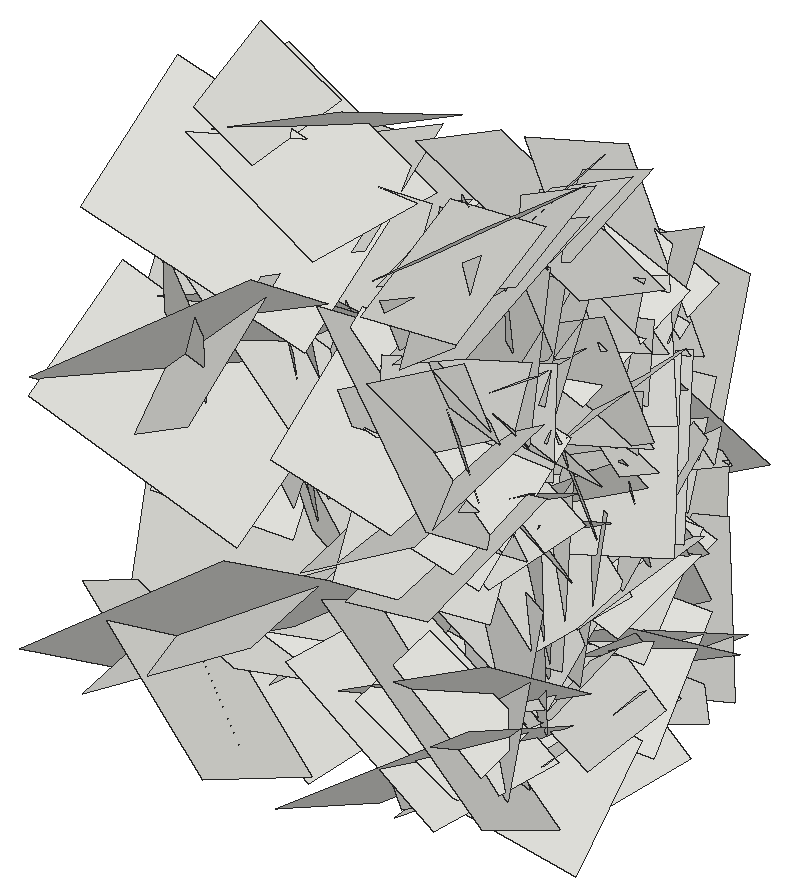
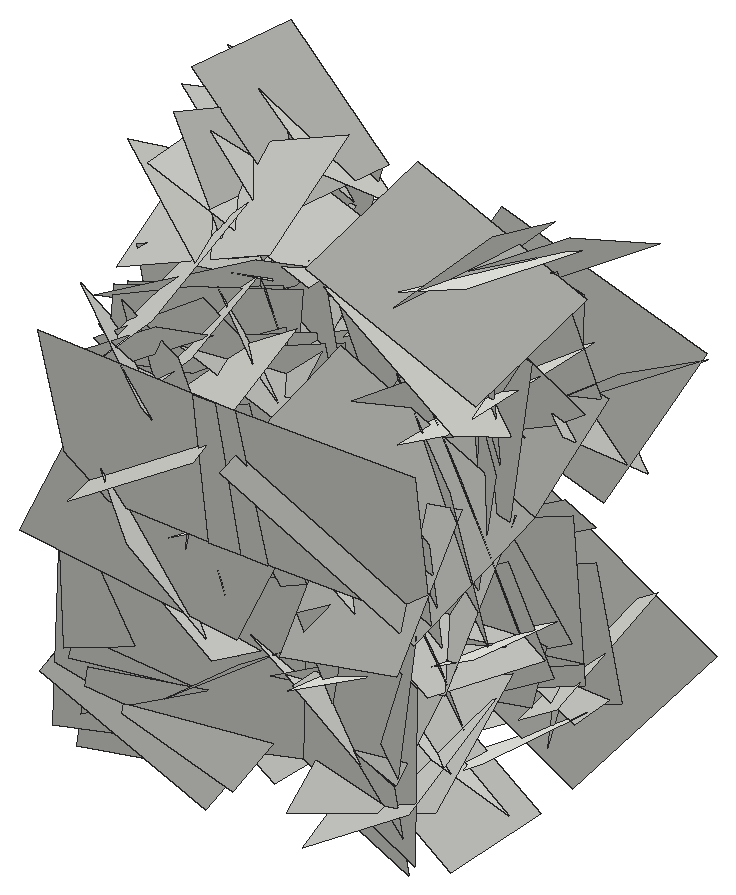
# SketchUp Ruby script. Lengths in inches.
U = 1.inch
M = Sketchup.active_model
def pt(a) = Geom::Point3d.new(a.map { |v| v * U })
def face(e, loops, mat)
  f = e.add_face(loops[0].map { |a| pt(a) })
  loops[1..].each { |l| e.add_face(l.map { |a| pt(a) }).erase! }
  f.material = f.back_material = mat if mat
  f
end
# faces: each face lists its corners as indices into pts; further lists are holes
def faces(e, pts, list, mat = nil) = list.each { |f| face(e, (f[0].is_a?(Array) ? f : [f]).map { |l| l.map { |i| pts[i] } }, mat) }
# xy, xz, yz: faces in a plane at the given z, y or x. An outline is a flat list of corners, or four numbers for a rectangle; further outlines are holes
def ring(l) = l.size == 4 ? [[l[0], l[1]], [l[2], l[1]], [l[2], l[3]], [l[0], l[3]]] : l.each_slice(2).to_a
def flat(e, list, mat, &to3) = list.each { |f| face(e, (f[0].is_a?(Array) ? f : [f]).map { |l| ring(l).map { |u, v| to3.(u, v) } }, mat) }
def xy(e, z, list, mat = nil) = flat(e, list, mat) { |x, y| [x, y, z] }
def xz(e, y, list, mat = nil) = flat(e, list, mat) { |x, z| [x, y, z] }
def yz(e, x, list, mat = nil) = flat(e, list, mat) { |y, z| [x, y, z] }
def lines(e, pts, list) = list.each { |a, b| e.add_line(pt(pts[a]), pt(pts[b])) }
# prism: a flat outline (further loops are holes) pulled along v
def prism(e, loops, v, mat = nil)
  f = face(e, loops, mat); d = Geom::Vector3d.new(v.map { |x| x * U })
  f.pushpull(f.normal.samedirection?(d) ? d.length : -d.length)
end
def box(e, o, s, mat = nil) = prism(e, [[o, [o[0] + s[0], o[1], o[2]], [o[0] + s[0], o[1] + s[1], o[2]], [o[0], o[1] + s[1], o[2]]]], [0, 0, s[2]], mat)
def at(x, y, z, deg = 0) = Geom::Transformation.translation(pt([x, y, z])) * Geom::Transformation.rotation(ORIGIN, Z_AXIS, deg.degrees)
def axes(o, x, y, z) = Geom::Transformation.new([*x, 0, *y, 0, *z, 0, *pt(o).to_a, 1])
def part(name) = M.definitions.add(name)
# library, detail: a bought-in or finely detailed component or shape, given as its bounding box
def library(name, o, s) = part(name).tap { |d| box(d.entities, o, s) }
def detail(e, o, s) = box(e.add_group.entities, o, s)
def put(e, d, t, mat = nil) = e.add_instance(d, t).tap { |i| i.material = mat if mat }
def group(e, t, mat = nil) = e.add_group.tap { |g| g.transformation = t; g.material = mat if mat }.entities
root = M.entities
c1 = part("Component\#6")
p = [[0.01,0,0],[0,3.24,4.54],[4.32,3.24,4.54],[4.33,0,0]]
faces(c1.entities,p,[[0,1,2,3]])
put(root,c1,axes([410.71,200.85,29.625],[-0.04324,0.39016,0.69087],[-0.10275,0.68414,-0.39209],[0.83473,0.10443,-0.01247]))
put(root,c1,axes([404.88,202.49,32.61],[0.11645,-0.17214,0.59947],[0.01233,0.60916,0.17278],[-0.661,-0.01896,0.10883]))
put(root,c1,axes([410.71,202.49,32.61],[-0.11645,-0.17214,0.59947],[-0.01233,0.60916,0.17278],[0.661,-0.01896,0.10883]))
put(root,c1,axes([400.91,199.54,32.72],[-0.14681,1.15124,0.44909],[-0.05729,0.44582,-1.15954],[1.30862,0.14867,-0.00039]))
put(root,c1,axes([414.68,199.54,32.72],[0.14681,1.15124,0.44909],[0.05729,0.44582,-1.15954],[-1.30862,0.14867,-0.00039]))
put(root,c1,axes([400.91,206.55,33.15],[0.00164,-0.95203,-0.71322],[-0.09471,-0.7113,0.94927],[1.25737,-0.05234,0.07244]))
put(root,c1,axes([414.68,206.55,33.15],[-0.00164,-0.95203,-0.71322],[0.09471,-0.7113,0.94927],[-1.25737,-0.05234,0.07244]))
put(root,c1,axes([410.71,202.42,34.22],[-0.03507,0.56649,-0.26791],[0.06705,-0.26389,-0.56581],[0.66085,0.05684,0.04319]))
put(root,c1,axes([410.71,205,37.54],[0.1597,-0.46751,-0.41946],[-0.05532,-0.43919,0.47075],[0.66349,0.07592,0.14021]))
put(root,c1,axes([400.91,204.59,30.02],[-0.04301,-1.09683,0.72238],[-0.12053,0.72294,1.0913],[1.38692,0.02882,0.11724]))
put(root,c1,axes([414.68,204.59,30.02],[0.04301,-1.09683,0.72238],[0.12053,0.72294,1.0913],[-1.38692,0.02882,0.11724]))
put(root,c1,axes([410.71,201.89,25.36],[0.12511,0.60489,0.30184],[-0.04372,0.31228,-0.60968],[0.71524,-0.08672,-0.09007]))
put(root,c1,axes([400.91,201.95,25.76],[0.02109,1.10253,-0.4508],[-0.04504,-0.44992,-1.10225],[1.2618,-0.03449,-0.03181]))
put(root,c1,axes([414.68,201.95,25.76],[-0.02109,1.10253,-0.4508],[0.04504,-0.44992,-1.10225],[-1.2618,-0.03449,-0.03181]))
put(root,c1,axes([414.68,200.125,30.08],[0.25415,0.9144,0.59243],[0.00684,0.60541,-0.93704],[-1.1549,0.20481,0.12483]))
put(root,c1,axes([400.91,205.99,22.98],[0.14358,-1.11124,-0.06865],[0.09474,-0.05808,1.11649],[1.17635,0.14031,-0.08154]))
put(root,c1,axes([414.68,205.99,22.98],[-0.14358,-1.11124,-0.06865],[-0.09474,-0.05808,1.11649],[-1.17635,0.14031,-0.08154]))
put(root,c1,axes([400.91,206.07,20.81],[-0.31441,-1.20333,0.63493],[-0.01893,0.65323,1.22967],[1.44208,-0.25378,0.15457]))
put(root,c1,axes([414.68,206.07,20.81],[0.31441,-1.20333,0.63493],[0.01893,0.65323,1.22967],[-1.44208,-0.25378,0.15457]))
put(root,c1,axes([414.68,201.41,38.375],[0.12316,0.77538,0.57304],[-0.12545,0.58429,-0.76661],[-1.01427,0.02189,0.1644]))
put(root,c1,axes([410.71,204.22,36.67],[0.08595,0.41822,-0.43473],[-0.01861,-0.43682,-0.42351],[0.63917,-0.06896,0.04613]))
put(root,c1,axes([410.71,204.95,35.05],[0.03568,0.1968,-0.61743],[-0.04358,-0.61637,-0.1987],[0.68554,-0.04943,0.01951]))
put(root,c1,axes([414.68,202.75,27.49],[0.17368,0.85862,-0.51485],[-0.1903,-0.48804,-0.87105],[-1.04401,0.2318,0.07312]))
put(root,c1,axes([410.71,202.89,32.22],[-0.0211,0.0618,0.84202],[-0.01452,0.84212,-0.06213],[0.89482,0.01512,0.01885]))
put(root,c1,axes([404.88,203.96,20.97],[-0.02025,-0.24988,0.58047],[0.03388,0.57961,0.25056],[-0.66903,0.03691,-0.00488]))
put(root,c1,axes([410.71,203.96,20.97],[0.02025,-0.24988,0.58047],[-0.03388,0.57961,0.25056],[0.66903,0.03691,-0.00488]))
put(root,c1,axes([410.71,202.23,33.91],[0.02493,0.60398,0.49928],[-0.17768,0.49182,-0.58706],[0.81142,0.08914,-0.14389]))
put(root,c1,axes([410.71,204.33,34.72],[-0.02793,-0.28222,0.66343],[0.05268,0.66158,0.28341],[0.7624,-0.05605,0.00473]))
put(root,c1,axes([414.68,207.21,30.03],[0.00943,-1.01637,-0.0193],[0.00822,-0.01923,1.01638],[-1.07752,-0.00904,0.00758]))
put(root,c1,axes([410.71,207.4,37.82],[-0.14382,-0.92009,0.02073],[-0.06912,0.03051,0.92748],[0.97309,-0.13382,0.06894]))
put(root,c1,axes([414.68,204.65,32.19],[-0.14144,0.68446,-0.34907],[-0.03425,-0.35898,-0.69154],[-0.81371,-0.10387,0.08978]))
put(root,c1,axes([400.91,201.85,37.73],[-0.10519,1.13817,0.58904],[-0.00109,0.59073,-1.14161],[1.35845,0.08861,0.0447]))
put(root,c1,axes([414.68,201.85,37.73],[0.10519,1.13817,0.58904],[0.00109,0.59073,-1.14161],[-1.35845,0.08861,0.0447]))
put(root,c1,axes([404.88,207.84,29.22],[0.13906,-0.51177,-0.49755],[-0.00544,-0.50655,0.51967],[-0.75658,-0.09042,-0.09518]))
put(root,c1,axes([410.71,207.84,29.22],[-0.13906,-0.51177,-0.49755],[0.00544,-0.50655,0.51967],[0.75658,-0.09042,-0.09518]))
put(root,c1,axes([410.71,206.625,39.5],[-0.00312,0.09172,-0.66161],[0.00201,-0.66161,-0.09173],[0.70801,0.00228,-0.00265]))
put(root,c1,axes([414.68,206.58,28.49],[-0.01093,-0.51913,0.63451],[-0.10311,0.63085,0.51456],[-0.86287,-0.06881,-0.06953]))
put(root,c1,axes([414.68,209.72,22.08],[0.18138,-0.91546,-0.54155],[0.07402,-0.53767,0.93095],[-1.12504,-0.18297,-0.02606]))
put(root,c1,axes([400.91,203.71,22.72],[-0.0324,0.32539,1.27516],[0.00551,1.27553,-0.32536],[1.39498,0.00251,0.0309]))
put(root,c1,axes([414.68,203.71,22.72],[0.0324,0.32539,1.27516],[-0.00551,1.27553,-0.32536],[-1.39498,0.00251,0.0309]))
put(root,c1,axes([414.68,204.07,39.0625],[0.02986,0.79051,0.40956],[-0.00815,0.40997,-0.79076],[-0.94369,0.02147,0.01979]))
put(root,c1,axes([400.91,207.91,30.98],[-0.03881,-0.77727,0.6188],[0.26695,0.59174,0.75817],[1.01873,-0.18467,-0.1751]))
put(root,c1,axes([414.68,207.91,30.98],[0.03881,-0.77727,0.6188],[-0.26695,0.59174,0.75817],[-1.01873,-0.18467,-0.1751]))
put(root,c1,axes([414.68,204.65,33.57],[-0.11682,0.36237,1.1463],[-0.15256,1.13885,-0.37385],[-1.26518,-0.17079,-0.06076]))
put(root,c1,axes([400.91,204.65,33.57],[0.11682,0.36237,1.1463],[0.15256,1.13885,-0.37385],[1.26518,-0.17079,-0.06076]))
put(root,c1,axes([400.91,205.05,35.75],[0.23328,1.34713,-0.22992],[0.05022,-0.24027,-1.36238],[1.44774,-0.20874,0.08431]))
put(root,c1,axes([414.68,205.05,35.75],[-0.23328,1.34713,-0.22992],[-0.05022,-0.24027,-1.36238],[-1.44774,-0.20874,0.08431]))
put(root,c1,axes([404.88,206,31.6],[0.1462,-0.08624,0.716],[0.07336,0.72719,0.07426],[-0.76092,0.05354,0.14472]))
put(root,c1,axes([410.71,206,31.6],[-0.1462,-0.08624,0.716],[-0.07336,0.72719,0.07426],[0.76092,0.05354,0.14472]))
put(root,c1,axes([414.68,209.27,26.87],[-0.02942,-0.98917,0.00062],[0.2303,-0.00549,0.9654],[-1.02292,0.02721,0.21733]))
put(root,c1,axes([414.68,205.35,34.65],[-0.12302,0.37909,0.72016],[0.00858,0.72795,-0.38188],[-0.86263,-0.04682,-0.1065]))
put(root,c1,axes([400.91,208.01,36.375],[-0.10923,0.38133,-1.06486],[0.05778,-1.06635,-0.38714],[1.19755,0.08623,-0.07845]))
put(root,c1,axes([414.68,208.01,36.375],[0.10923,0.38133,-1.06486],[-0.05778,-1.06635,-0.38714],[-1.19755,0.08623,-0.07845]))
put(root,c1,axes([414.68,205.67,24.52],[-0.15369,0.87531,0.08009],[0.01982,0.08422,-0.88666],[-0.9315,-0.14262,-0.03208]))
put(root,c1,axes([400.91,209.74,33.23],[0.15201,0.07034,-1.21602],[-0.20156,-1.20811,-0.09231],[1.2753,-0.19933,0.13035]))
put(root,c1,axes([414.68,209.74,33.23],[-0.15201,0.07034,-1.21602],[0.20156,-1.20811,-0.09231],[-1.2753,-0.19933,0.13035]))
put(root,c1,axes([400.91,205.63,39.17],[0.17317,1.06099,0.10432],[0.22006,0.07185,-1.05594],[1.10844,-0.18002,0.19334]))
put(root,c1,axes([414.68,205.63,39.17],[-0.17317,1.06099,0.10432],[-0.22006,0.07185,-1.05594],[-1.10844,-0.18002,0.19334]))
put(root,c1,axes([400.91,205.38,23.16],[0.04798,1.09948,0.05597],[0.01409,0.05547,-1.10036],[1.16688,-0.04588,0.01099]))
put(root,c1,axes([414.68,205.38,23.16],[-0.04798,1.09948,0.05597],[-0.01409,0.05547,-1.10036],[-1.16688,-0.04588,0.01099]))
put(root,c1,axes([404.88,208.95,27.68],[0.1117,0.11156,-0.75397],[0.06454,-0.75994,-0.10393],[-0.80532,-0.04543,-0.11291]))
put(root,c1,axes([410.71,208.95,27.68],[-0.1117,0.11156,-0.75397],[-0.06454,-0.75994,-0.10393],[0.80532,-0.04543,-0.11291]))
put(root,c1,axes([400.91,205.46,24.09],[0.08024,0.04196,1.34674],[-0.06239,1.34768,-0.03868],[1.42687,0.05657,-0.07742]))
put(root,c1,axes([414.68,205.46,24.09],[-0.08024,0.04196,1.34674],[0.06239,1.34768,-0.03868],[-1.42687,0.05657,-0.07742]))
put(root,c1,axes([404.88,210.37,37.54],[0.0852,-0.7988,-0.26142],[0.21653,-0.23617,0.78446],[-0.8642,-0.13792,0.17078]))
put(root,c1,axes([410.71,210.37,37.54],[-0.0852,-0.7988,-0.26142],[-0.21653,-0.23617,0.78446],[0.8642,-0.13792,0.17078]))
put(root,c1,axes([400.91,205.46,33.43],[0.14097,0.63084,0.7943],[-0.06243,0.80455,-0.62912],[1.07339,-0.03606,-0.14091]))
put(root,c1,axes([414.68,205.46,33.43],[-0.14097,0.63084,0.7943],[0.06243,0.80455,-0.62912],[-1.07339,-0.03606,-0.14091]))
put(root,c1,axes([400.91,211.43,33.78],[-0.23599,-0.36182,-1.29322],[-0.09706,-1.30373,0.38052],[1.42014,-0.14923,-0.18889]))
put(root,c1,axes([414.68,211.43,33.78],[0.23599,-0.36182,-1.29322],[0.09706,-1.30373,0.38052],[-1.42014,-0.14923,-0.18889]))
put(root,c1,axes([410.71,206.77,29.69],[0.13468,0.0618,0.68245],[-0.14259,0.68282,-0.03679],[0.71222,0.12502,-0.13642]))
put(root,c1,axes([410.71,209.27,26.93],[0.01951,-0.6006,0.29742],[0.06663,0.29777,0.59742],[0.70729,-0.01148,-0.06448]))
put(root,c1,axes([400.91,205.51,24.88],[0.13882,1.11155,0.63897],[0.19603,0.6192,-1.11507],[1.34484,-0.205,0.09658]))
put(root,c1,axes([414.68,205.51,24.88],[-0.13882,1.11155,0.63897],[-0.19603,0.6192,-1.11507],[-1.34484,-0.205,0.09658]))
put(root,c1,axes([414.68,211.47,22.62],[0.20513,-1.22241,0.07319],[0.04122,0.08019,1.23659],[-1.29742,-0.19072,0.05085]))
put(root,c1,axes([400.91,206.12,25.83],[0.28838,0.48251,1.20317],[0.13396,1.21365,-0.51529],[1.36755,-0.22063,-0.20324]))
put(root,c1,axes([414.68,206.12,25.83],[-0.28838,0.48251,1.20317],[-0.13396,1.21365,-0.51529],[-1.36755,-0.22063,-0.20324]))
put(root,c1,axes([414.68,210.75,36.02],[0.14272,-1.0645,0.43866],[-0.22696,0.41079,1.0626],[-1.19913,-0.20445,-0.14891]))
put(root,c1,axes([400.91,210.75,36.02],[-0.14272,-1.0645,0.43866],[0.22696,0.41079,1.0626],[1.19913,-0.20445,-0.14891]))
put(root,c1,axes([400.91,208.81,31.45],[-0.04602,0.84125,-1.04893],[-0.18208,-1.04435,-0.83047],[1.4136,-0.10713,-0.14111]))
put(root,c1,axes([414.68,208.81,31.45],[0.04602,0.84125,-1.04893],[0.18208,-1.04435,-0.83047],[-1.4136,-0.10713,-0.14111]))
put(root,c1,axes([410.71,209.37,33.75],[-0.00852,0.3462,-0.76666],[-0.09329,-0.76284,-0.34355],[0.88678,-0.07692,-0.04351]))
put(root,c1,axes([410.71,207.43,34.16],[0.11276,0.04323,0.70746],[-0.03845,0.71477,-0.03823],[0.75032,0.03013,-0.10828]))
put(root,c1,axes([400.91,211.99,33.59],[-0.13241,-0.25962,-1.28668],[-0.09489,-1.2878,0.26854],[1.38813,-0.1128,-0.10438]))
put(root,c1,axes([414.68,211.99,33.59],[0.13241,-0.25962,-1.28668],[0.09489,-1.2878,0.26854],[-1.38813,-0.1128,-0.10438]))
put(root,c1,axes([414.68,210.23,35.31],[-0.06568,0.00099,-0.81141],[-0.08224,-0.81005,0.00494],[-0.85616,0.07773,0.06177]))
put(root,c1,axes([414.68,206.36,33.23],[0.09168,1.1059,0.20164],[0.04784,0.19866,-1.1089],[-1.19063,0.09314,-0.02903]))
put(root,c1,axes([410.71,207.11,31.75],[-0.23783,0.22127,0.93353],[-0.03566,0.95632,-0.23476],[1.01634,0.08533,0.21022]))
put(root,c1,axes([400.91,211.92,20.51],[0.20622,-1.25394,-0.15944],[-0.06822,-0.17093,1.26581],[1.33814,0.18453,0.0891]))
put(root,c1,axes([414.68,211.92,20.51],[-0.20622,-1.25394,-0.15944],[0.06822,-0.17093,1.26581],[-1.33814,0.18453,0.0891]))
put(root,c1,axes([400.91,211.85,35.53],[0.11979,-0.95717,-0.48165],[0.13908,-0.46832,0.96146],[1.12727,0.15949,-0.06744]))
put(root,c1,axes([414.68,211.85,35.53],[-0.11979,-0.95717,-0.48165],[-0.13908,-0.46832,0.96146],[-1.12727,0.15949,-0.06744]))
put(root,c1,axes([414.68,210.61,30.96],[-0.02538,-1.03384,0.49264],[0.2847,0.47394,1.00764],[-1.18007,0.13657,0.23251]))
put(root,c1,axes([410.71,211.91,37.97],[-0.10192,-0.72839,-0.40458],[-0.00784,-0.4065,0.73361],[0.88316,-0.08767,-0.04018]))
put(root,c1,axes([400.91,206.95,24.98],[0.09414,0.39654,1.07266],[-0.12922,1.07305,-0.38659],[1.20532,0.08407,-0.12522]))
put(root,c1,axes([414.68,206.95,24.98],[-0.09414,0.39654,1.07266],[0.12922,1.07305,-0.38659],[-1.20532,0.08407,-0.12522]))
put(root,c1,axes([400.91,206.8125,26.89],[-0.15204,1.11982,0.24611],[0.19339,0.26716,-1.10927],[1.19986,0.09884,0.20998]))
put(root,c1,axes([414.68,206.8125,26.89],[0.15204,1.11982,0.24611],[-0.19339,0.26716,-1.10927],[-1.19986,0.09884,0.20998]))
put(root,c1,axes([400.91,213.06,27.02],[-0.109,-1.16412,-0.17966],[0.1638,-0.19212,1.15639],[1.23778,-0.07709,-0.16885]))
put(root,c1,axes([414.68,213.06,27.02],[0.109,-1.16412,-0.17966],[-0.1638,-0.19212,1.15639],[-1.23778,-0.07709,-0.16885]))
put(root,c1,axes([400.91,212.41,27.7],[0.11035,-0.46639,-0.85158],[-0.0233,-0.85737,0.46687],[1.02892,0.03061,0.1019]))
put(root,c1,axes([414.68,212.41,27.7],[-0.11035,-0.46639,-0.85158],[0.0233,-0.85737,0.46687],[-1.02892,0.03061,0.1019]))
put(root,c1,axes([400.91,212.85,24.81],[-0.10314,-0.72888,-0.73382],[0.20394,-0.73695,0.70648],[1.07722,0.06973,-0.20401]))
put(root,c1,axes([414.68,212.85,24.81],[0.10314,-0.72888,-0.73382],[-0.20394,-0.73695,0.70648],[-1.07722,0.06973,-0.20401]))
put(root,c1,axes([410.71,209.14,33.82],[0.16184,0.36707,0.52708],[-0.01835,0.54392,-0.37378],[0.68059,-0.07262,-0.13541]))
put(root,c1,axes([410.71,212.36,26.625],[-0.06935,-0.64087,-0.11796],[0.11905,-0.12787,0.63241],[0.68039,-0.04294,-0.12268]))
put(root,c1,axes([400.91,208.94,26.04],[-0.1299,1.02121,-0.60997],[0.25035,-0.5801,-1.01865],[1.23578,0.22487,0.14225]))
put(root,c1,axes([414.68,208.94,26.04],[0.1299,1.02121,-0.60997],[-0.25035,-0.5801,-1.01865],[-1.23578,0.22487,0.14225]))
put(root,c1,axes([414.68,210.17,27.25],[-0.0389,-0.19659,0.74237],[-0.03773,0.74285,0.19496],[-0.81316,-0.02506,-0.04456]))
put(root,c1,axes([400.91,209.77,25.57],[-0.04769,1.02209,-0.46416],[-0.05126,-0.46587,-1.02116],[1.18879,0.02092,-0.06265]))
put(root,c1,axes([414.68,209.77,25.57],[0.04769,1.02209,-0.46416],[0.05126,-0.46587,-1.02116],[-1.18879,0.02092,-0.06265]))
put(root,c1,axes([414.68,212.48,33.12],[-0.02538,-1.03384,0.49264],[0.2847,0.47394,1.00764],[-1.18007,0.13657,0.23251]))
put(root,c1,axes([400.91,211.63,27.44],[0.13698,0.50835,-0.7639],[0.02564,-0.77306,-0.51036],[0.97231,-0.05123,0.12108]))
put(root,c1,axes([414.68,211.63,27.44],[-0.13698,0.50835,-0.7639],[-0.02564,-0.77306,-0.51036],[-0.97231,-0.05123,0.12108]))
put(root,c1,axes([400.91,212.99,32.26],[0.05541,-0.21084,-0.92918],[0.15034,-0.91849,0.21639],[0.99872,0.14996,0.01898]))
put(root,c1,axes([414.68,212.99,32.26],[-0.05541,-0.21084,-0.92918],[-0.15034,-0.91849,0.21639],[-0.99872,0.14996,0.01898]))
put(root,c1,axes([410.71,212.78,35.18],[-0.06835,-0.19577,-0.64021],[0.13077,-0.63563,0.18195],[0.69749,0.09999,-0.09685]))
put(root,c1,axes([400.91,213.71,29.11],[-0.07729,-1.24842,0.49404],[-0.03127,0.49613,1.24937],[1.42283,-0.05691,0.0543]))
put(root,c1,axes([414.68,213.71,29.11],[0.07729,-1.24842,0.49404],[0.03127,0.49613,1.24937],[-1.42283,-0.05691,0.0543]))
put(root,c1,axes([400.91,213.59,29.33],[0.10669,0.07311,-1.12569],[-0.06812,-1.12796,-0.079],[1.19381,-0.0709,0.09609]))
put(root,c1,axes([414.68,213.59,29.33],[-0.10669,0.07311,-1.12569],[0.06812,-1.12796,-0.079],[-1.19381,-0.0709,0.09609]))
put(root,c1,axes([400.91,213.57,27.56],[-0.01798,0.03957,-1.39555],[0.22262,-1.3797,-0.04168],[1.46303,0.21042,-0.01081]))
put(root,c1,axes([414.68,213.57,27.56],[0.01798,0.03957,-1.39555],[-0.22262,-1.3797,-0.04168],[-1.46303,0.21042,-0.01081]))
put(root,c1,axes([400.91,211.375,32.78],[-0.08242,0.8278,-0.94283],[0.12426,-0.93571,-0.83122],[1.32412,0.13934,0.01932]))
put(root,c1,axes([414.68,211.375,32.78],[0.08242,0.8278,-0.94283],[-0.12426,-0.93571,-0.83122],[-1.32412,0.13934,0.01932]))
put(root,c1,axes([404.88,210.56,30.82],[0.08988,0.23539,0.56706],[-0.00516,0.57268,-0.23699],[-0.65079,0.02797,0.0802]))
put(root,c1,axes([410.71,210.56,30.82],[-0.08988,0.23539,0.56706],[0.00516,0.57268,-0.23699],[0.65079,0.02797,0.0802]))
put(root,c1,axes([414.68,208.86,27.22],[0.22907,0.58895,0.94038],[0.09031,0.94642,-0.61231],[-1.17269,0.18793,0.13653]))
put(root,c1,axes([404.88,211.4,20.36],[0.11841,0.02386,0.67628],[-0.07272,0.6823,-0.01274],[-0.7136,-0.06557,0.11352]))
put(root,c1,axes([410.71,211.4,20.36],[-0.11841,0.02386,0.67628],[0.07272,0.6823,-0.01274],[0.7136,-0.06557,0.11352]))
put(root,c1,axes([410.71,211.1,35.2],[0.07899,0.5337,0.27791],[0.02897,0.27674,-0.53878],[0.63716,-0.07875,-0.00996]))
put(root,c1,axes([414.68,210.92,34.25],[-0.13403,0.53039,0.57824],[0.04314,0.58935,-0.53168],[-0.83061,-0.05497,-0.12092]))
put(root,c1,axes([400.56,214.11,35.21],[0.07772,-0.27644,-1.33377],[0.91911,-1.02064,0.2592],[1.11351,0.86175,-0.12086]))
put(root,c1,axes([415.03,214.11,35.21],[-0.07772,-0.27644,-1.33377],[-0.91911,-1.02064,0.2592],[-1.11351,0.86175,-0.12086]))
